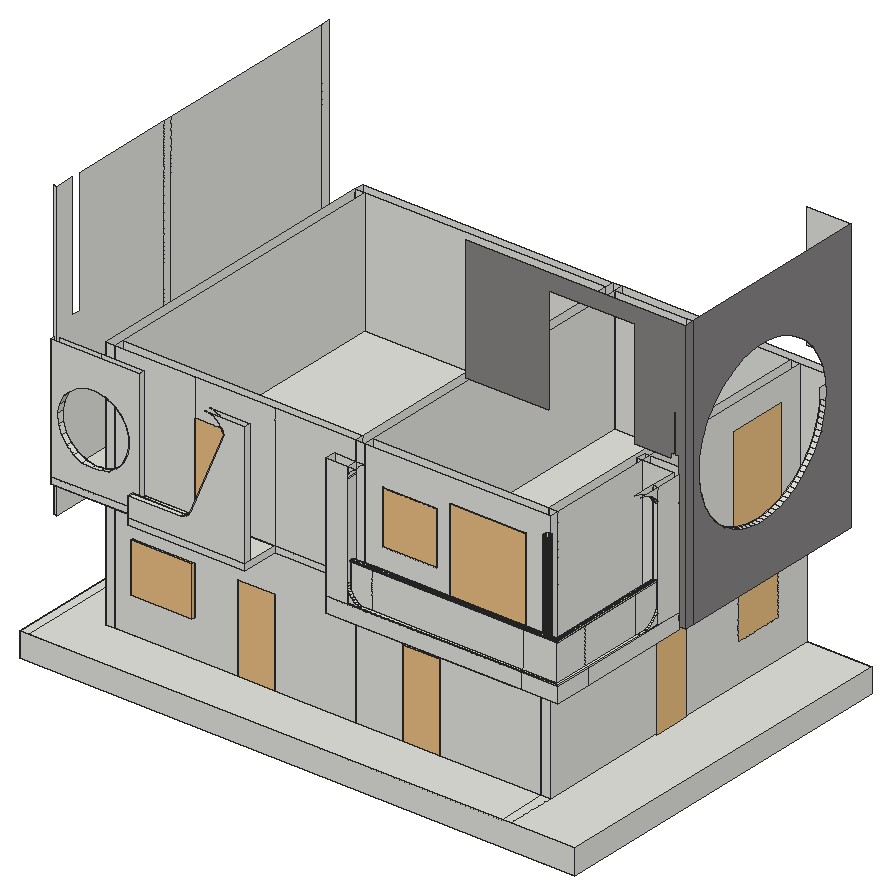
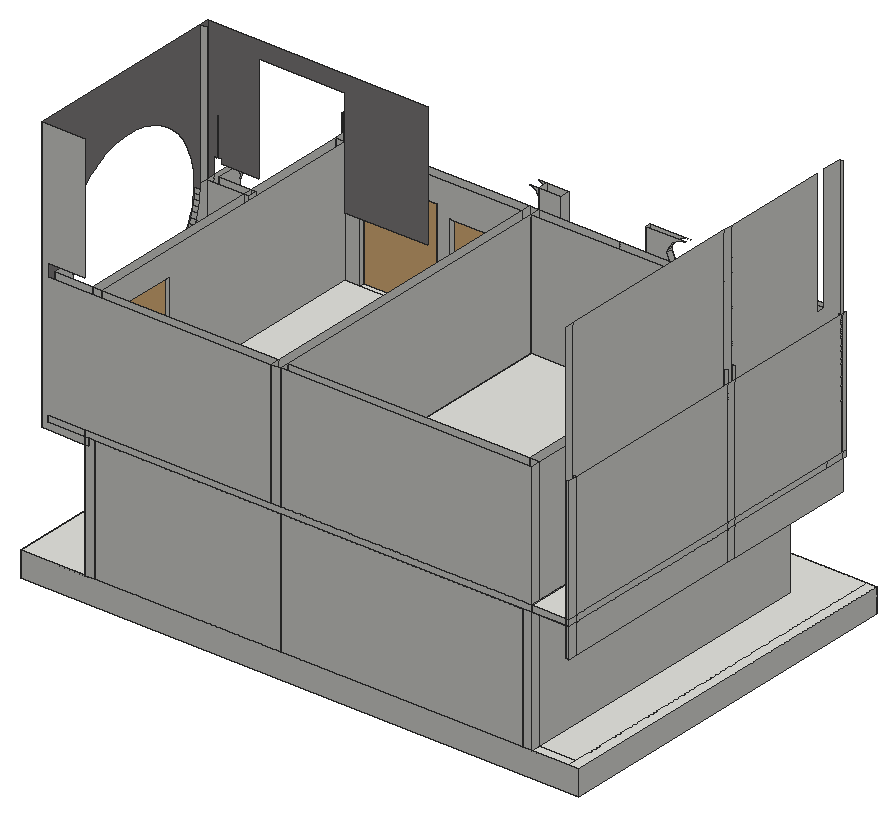
# SketchUp Ruby script. Lengths in inches.
U = 1.inch
M = Sketchup.active_model
def pt(a) = Geom::Point3d.new(a.map { |v| v * U })
def face(e, loops, mat)
  f = e.add_face(loops[0].map { |a| pt(a) })
  loops[1..].each { |l| e.add_face(l.map { |a| pt(a) }).erase! }
  f.material = f.back_material = mat if mat
  f
end
# faces: each face lists its corners as indices into pts; further lists are holes
def faces(e, pts, list, mat = nil) = list.each { |f| face(e, (f[0].is_a?(Array) ? f : [f]).map { |l| l.map { |i| pts[i] } }, mat) }
# xy, xz, yz: faces in a plane at the given z, y or x. An outline is a flat list of corners, or four numbers for a rectangle; further outlines are holes
def ring(l) = l.size == 4 ? [[l[0], l[1]], [l[2], l[1]], [l[2], l[3]], [l[0], l[3]]] : l.each_slice(2).to_a
def flat(e, list, mat, &to3) = list.each { |f| face(e, (f[0].is_a?(Array) ? f : [f]).map { |l| ring(l).map { |u, v| to3.(u, v) } }, mat) }
def xy(e, z, list, mat = nil) = flat(e, list, mat) { |x, y| [x, y, z] }
def xz(e, y, list, mat = nil) = flat(e, list, mat) { |x, z| [x, y, z] }
def yz(e, x, list, mat = nil) = flat(e, list, mat) { |y, z| [x, y, z] }
def lines(e, pts, list) = list.each { |a, b| e.add_line(pt(pts[a]), pt(pts[b])) }
# prism: a flat outline (further loops are holes) pulled along v
def prism(e, loops, v, mat = nil)
  f = face(e, loops, mat); d = Geom::Vector3d.new(v.map { |x| x * U })
  f.pushpull(f.normal.samedirection?(d) ? d.length : -d.length)
end
def box(e, o, s, mat = nil) = prism(e, [[o, [o[0] + s[0], o[1], o[2]], [o[0] + s[0], o[1] + s[1], o[2]], [o[0], o[1] + s[1], o[2]]]], [0, 0, s[2]], mat)
def at(x, y, z, deg = 0) = Geom::Transformation.translation(pt([x, y, z])) * Geom::Transformation.rotation(ORIGIN, Z_AXIS, deg.degrees)
def axes(o, x, y, z) = Geom::Transformation.new([*x, 0, *y, 0, *z, 0, *pt(o).to_a, 1])
def part(name) = M.definitions.add(name)
# library, detail: a bought-in or finely detailed component or shape, given as its bounding box
def library(name, o, s) = part(name).tap { |d| box(d.entities, o, s) }
def detail(e, o, s) = box(e.add_group.entities, o, s)
def put(e, d, t, mat = nil) = e.add_instance(d, t).tap { |i| i.material = mat if mat }
def group(e, t, mat = nil) = e.add_group.tap { |g| g.transformation = t; g.material = mat if mat }.entities
root = M.entities
M.materials.add("[Brick Tumbled]").color = [135, 132, 132]
c1 = library("Door 243 053",[-21.6,-2.79,-0.07],[43.2,5.58,82.64])
c2 = library("Window 46-08",[-34.875,-3.16,0],[69.74,4.26,70.87])
c3 = library("Window 46-47",[-61.02,-2.17,0],[122.04,4.34,74.02])
xy(root,-24,[[0,0,539.56,360]])
xy(root,0,[[0,0,9,360],[9,0,468,0,468,48,369.625,48,369.625,57,333.625,57,333.625,48,209.125,48,209.125,57,173.125,57,173.125,48,45,48,45,351,9,351],[468,0,477,48],[477,0,539.56,360],[45,48,54,360],
  [54,48,173.125,57],[209.125,48,288,57],[288,48,333.625,57],[369.625,48,468,57],[468,48,477,176.1875],
  [54,57,150,351],[150,57,159,351],[150,57,279,351],[159,57,279,351],[279,57,288,351],
  [288,57,468,351],[468,176.1875,477,212.1875],[468,212.1875,477,360],[9,351,45,360],[54,351,288,360],
  [288,351,468,360]])
xy(root,36,[[71,48,131,57],[468,276,477,324]])
xy(root,84,[[71,48,131,57],[173.125,48,209.125,57],[333.625,48,369.625,57],[468,176.1875,477,212.1875],[468,276,477,324]])
xy(root,91.5625,[[9,29.25,12.34,159.3125],[9,159.3125,12.34,168.3125],[9,168.3125,12.34,351],[9,351,12.34,360]])
xy(root,111.125,[[288,12,468,17.99],[468,12,477,17.99],[477,12,513,17.99],[509.76,17.99,513,48],[509.76,48,513,159.3125]])
xy(root,113.5,[[473.9375,159.3125,519.125,168.3125],[513,168.3125,513,351,473.75,351,473.75,360,519.125,360,519.125,168.3125]],"[Brick Tumbled]")
xy(root,120,[[95.3125,12,95.3125,25.8125,131,25.8125,131,48,209.125,48,209.125,12],[288,17.99,468,48],[468,17.99,477,48],[477,17.99,509.76,48],[9,25.8125,54,48],
  [54,25.8125,131,48],[9,48,45,351],[45,48,54,360],[54,48,288,57],[288,48,468,57],
  [468,48,477,48,477,159.3125,473.9375,159.3125,473.9375,168.3125,477,168.3125,477,351,473.75,351,473.75,360,468,360],[477,48,509.76,159.3125],[54,57,150,351],[150,57,159,351],[150,57,279,351],
  [279,57,288,351],[288,57,468,351],[473.9375,159.3125,477,168.3125],[477,159.3125,513,168.3125],[477,168.3125,513,351],
  [9,351,45,360],[54,351,288,360],[288,351,468,360],[473.75,351,477,360],[477,351,513,360]])
xy(root,126,[[95.3125,12,209.125,17.48],[288,12,308.6875,21.82],[308.6875,12,327.12,19.52],[327.12,12,327.12,19.52,505.48,19.52,505.48,159.3125,507.74,159.3125,507.74,112.72,513,112.72,513,12],[95.3125,17.48,209.125,17.48,209.125,48,131,48,131,25.8125,95.3125,25.8125],
  [[327.12,19.52,505.48,19.52,505.48,159.3125,477,159.3125,477,48,288,48,288,21.82,327.12,21.82],[493.53,20.08,492.64,20.28,491.83,20.7,491.16,21.32,490.67,22.09,490.39,22.96,490.35,23.875,490.55,24.77,490.98,25.58,491.59,26.25,492.37,26.74,493.24,27.01,494.15,27.05,495.04,26.85,495.85,26.43,496.52,25.8125,497.01,25.04,497.29,24.17,497.33,23.25,497.125,22.36,496.7,21.55,496.09,20.88,495.3125,20.39,494.44,20.12]],[308.6875,19.52,327.12,21.82],[493.53,20.08,492.64,20.28,491.83,20.7,491.16,21.32,490.67,22.09,490.39,22.96,490.35,23.875,490.55,24.77,490.98,25.58,491.59,26.25,492.37,26.74,493.24,27.01,494.15,27.05,495.04,26.85,495.85,26.43,496.52,25.8125,497.01,25.04,497.29,24.17,497.33,23.25,497.125,22.36,496.7,21.55,496.09,20.88,495.3125,20.39,494.44,20.12],[9,25.8125,54,31.1875],[54,25.8125,95.3125,31.1875],
  [95.3125,25.8125,131,25.8125,131,48,54,48,54,31.1875,95.3125,31.1875],[9,31.1875,54,48],[9,48,45,360],[45,48,54,351],[54,48,131,57],
  [131,48,173.125,57],[173.125,48,288,57],[288,48,297,360],[297,48,379.04,57],[379.04,48,453.36,57],
  [453.36,48,477,57],[54,57,288,351],[297,57,468,351],[468,57,468,269.23,477,269.23,477,168.3125,472.375,168.3125,472.375,159.3125,477,159.3125,477,57],[507.74,112.72,513,134.0625],
  [507.74,134.0625,513,134.0625,513,168.3125,477,168.3125,477,159.3125,507.74,159.3125],[472.375,159.3125,477,168.3125],[477,168.3125,513,351],[468,269.23,477,328.73],[468,328.73,477,351],
  [45,351,288,360],[297,351,477,360],[477,351,513,360]])
xy(root,127.25,[[308.6875,12,327.12,12,327.12,14.75,309.62,14.75,309.62,16.77,327.12,16.77,327.12,19.52,308.6875,19.52],[327.12,12,513,12,513,112.72,510.25,112.72,510.25,14.75,327.12,14.75],[309.62,14.75,327.12,16.77],[327.12,14.75,329.87,16.77],[329.87,14.75,329.87,16.77,508.23,16.77,508.23,109.97,510.25,109.97,510.25,14.75],
  [327.12,16.77,508.23,16.77,508.23,112.72,507.74,112.72,507.74,159.3125,505.48,159.3125,505.48,19.52,327.12,19.52],[508.23,109.97,510.25,112.72],[507.74,112.72,508.23,134.0625],[508.23,112.72,510.25,134.0625],[510.25,112.72,513,134.0625]])
xy(root,145.31,[[95.3125,12,145.3,17.48]])
xy(root,162.59,[[314.49,48,366.36,57]])
xy(root,163.25,[[[308.44,13.58,308.44,17.9375,507.0625,17.9375,507.0625,135.23,511.42,135.23,511.42,13.58],[309.62,14.75,510.25,14.75,510.25,134.0625,508.23,134.0625,508.23,16.77,309.62,16.77]],[309.62,14.75,309.62,16.77,508.23,16.77,508.23,134.0625,510.25,134.0625,510.25,14.75]])
xy(root,164.125,[[[308.44,13.58,511.42,13.58,511.42,135.23,507.0625,135.23,507.0625,17.9375,308.44,17.9375],[309.62,14.75,309.62,16.77,508.23,16.77,508.23,134.0625,510.25,134.0625,510.25,14.75]],[309.62,14.75,510.25,14.75,510.25,134.0625,508.23,134.0625,508.23,16.77,309.62,16.77]])
xy(root,210,[[131,48,173.125,57]])
xy(root,214.46,[[314.49,48,366.36,57]])
xy(root,222.27,[[468,269.23,477,328.73]])
xy(root,223.3125,[[379.04,48,453.36,57]])
xz(root,0,[[0,-24,539.56,0]])
xz(root,12,[[288,111.125,477,126],[477,111.125,513,126],[95.3125,120,209.125,126],[95.3125,126,209.125,126,209.125,246,170.0625,246,172.1875,245.88,174.28,245.51,176.32,244.91,178.28,244.08,180.13,243.03,181.84,241.77,183.41,240.33,184.79,238.71,185.98,236.95,186.96,235.07,187.72,233.08,188.25,231.02,155.44,151.72,154.86,150.87,154.22,150.06,153.52,149.29,152.77,148.59,151.96,147.94,151.11,147.36,150.21,146.84,149.28,146.38,148.32,146,147.33,145.7,146.32,145.46,145.3,145.31,95.3125,145.31],[288,126,308.6875,246],
  [308.6875,126,327.12,126,324.71,126.16,322.35,126.63,320.51,127.25,308.6875,127.25],[327.12,126,327.12,127.25,320.51,127.25,322.35,126.63,324.71,126.16],[327.12,126,477,127.25],[477,126,513,127.25],[308.6875,127.25,320.51,127.25,320.0625,127.4,317.9,128.47,315.9,129.81,314.09,131.4,312.5,133.21,311.16,135.21,310.09,137.375,309.32,139.66,308.85,142.02,308.6875,144.43],
  [308.6875,235.27,308.76,236.49,308.96,237.7,309.3,238.88,309.76,240.02,310.35,241.1,311.06,242.1,311.87,243.02,312.78,243.85,313.77,244.5625,314.84,245.17,315.97,245.65,317.15,246,308.6875,246]])
xz(root,13.58,[[308.44,163.25,329.87,164.125],[329.87,163.25,477,164.125],[477,163.25,511.42,164.125]])
xz(root,14.75,[[309.62,127.25,329.87,163.25],[329.87,127.25,477,163.25],[477,127.25,510.25,163.25],[309.62,163.25,329.87,164.125],[329.87,163.25,477,164.125],
  [477,163.25,510.25,164.125]])
xz(root,16.77,[[309.62,127.25,329.87,163.25],[329.87,127.25,477,163.25],[477,127.25,508.23,163.25],[309.62,163.25,329.87,164.125],[329.87,163.25,477,164.125],
  [477,163.25,508.23,164.125]])
xz(root,17.48,[[95.3125,126,95.3125,145.31,145.3,145.31,146.32,145.46,147.33,145.7,148.32,146,149.28,146.38,150.21,146.84,151.11,147.36,151.96,147.94,152.77,148.59,153.52,149.29,154.22,150.06,154.86,150.87,155.44,151.72,188.25,231.02,187.72,233.08,186.96,235.07,185.98,236.95,184.79,238.71,183.41,240.33,181.84,241.77,180.13,243.03,178.28,244.08,176.32,244.91,174.28,245.51,172.1875,245.88,170.0625,246,209.125,246,209.125,126]])
xz(root,17.9375,[[308.44,163.25,329.87,164.125],[329.87,163.25,477,164.125],[477,163.25,507.0625,164.125]])
xz(root,17.99,[[288,111.125,468,120],[468,111.125,477,120],[477,111.125,509.76,120]])
xz(root,19.52,[[308.6875,126,327.12,127.25],[327.12,126,477,127.25],[477,126,505.48,127.25]])
xz(root,21.82,[[288,126,308.6875,246],[308.6875,126,308.6875,144.43,308.85,142.02,309.32,139.66,310.09,137.375,311.16,135.21,312.5,133.21,314.09,131.4,315.9,129.81,317.9,128.47,320.0625,127.4,322.35,126.63,324.71,126.16,327.12,126],[308.6875,235.27,308.6875,246,317.15,246,315.97,245.65,314.84,245.17,313.77,244.5625,312.78,243.85,311.87,243.02,311.06,242.1,310.35,241.1,309.76,240.02,309.3,238.88,308.96,237.7,308.76,236.49]])
xz(root,25.8125,[[9,120,95.3125,126],[95.3125,120,131,126],[[9,126,95.3125,246],[48.3125,147.1,39.51,148.92,31.48,152.96,24.77,158.94,19.84,166.46,17.02,175,16.5,183.97,18.33,192.77,22.37,200.8,28.35,207.52,35.86,212.45,44.4,215.27,53.375,215.78,62.18,213.96,70.21,209.92,76.92,203.9375,81.85,196.42,84.67,187.88,85.1875,178.91,83.36,170.11,79.32,162.08,73.34,155.37,65.83,150.43,57.29,147.61]]])
xz(root,29.25,[[9,91.5625,12.34,378]])
xz(root,31.1875,[[9,126,9,246,54,246,54,215.66,53.375,215.78,44.4,215.27,35.86,212.45,28.35,207.52,22.37,200.8,18.33,192.77,16.5,183.97,17.02,175,19.84,166.46,24.77,158.94,31.48,152.96,39.51,148.92,48.3125,147.1,54,147.42,54,126],[54,126,54,147.42,57.29,147.61,65.83,150.43,73.34,155.37,79.32,162.08,83.36,170.11,85.1875,178.91,84.67,187.88,81.85,196.42,76.92,203.9375,70.21,209.92,62.18,213.96,54,215.66,54,246,95.3125,246,95.3125,126]])
xz(root,48,[[45,0,54,120],[[54,0,173.125,0,173.125,84,209.125,84,209.125,0,288,0,288,120,54,120],[71,36,131,84]],[288,0,333.625,0,333.625,84,369.625,84,369.625,0,468,0,468,120,288,120],[468,0,477,120],[9,120,45,126],
  [131,120,209.125,126],[209.125,120,288,126],[288,120,477,126],[45,126,54,246],[54,126,131,246],
  [173.125,126,209.125,126,209.125,246,131,246,131,210,173.125,210],[209.125,126,288,246],[288,126,297,246],[[297,126,379.04,126,379.04,223.3125,453.36,223.3125,453.36,126,477,126,477,246,297,246],[314.49,162.59,366.36,214.46]]])
xz(root,57,[[[54,0,150,120],[71,36,131,84]],[150,0,159,120],[159,0,159,120,279,120,279,0,209.125,0,209.125,84,173.125,84,173.125,0],[279,0,288,120],[288,0,288,120,468,120,468,0,369.625,0,369.625,84,333.625,84,333.625,0],
  [54,126,54,246,288,246,288,126,173.125,126,173.125,210,131,210,131,126],[[297,126,297,246,468,246,468,126,453.36,126,453.36,223.3125,379.04,223.3125,379.04,126],[314.49,162.59,366.36,214.46]],[468,126,477,246]])
xz(root,112.72,[[507.74,126,513,127.25]])
xz(root,134.0625,[[507.74,127.25,508.23,139.33],[508.23,127.25,510.25,139.33],[510.25,127.25,513,139.33],[507.74,139.33,508.23,139.33,508.23,164.125,510.25,164.125,510.25,139.33,513,139.33,513,231.76,507.74,231.76],[508.23,139.33,510.25,163.25],
  [508.23,163.25,510.25,164.125],[507.74,231.76,513,246]])
xz(root,135.23,[[507.0625,163.25,511.42,164.125]])
xz(root,159.3125,[[9,91.5625,12.34,258],[509.76,111.125,513,113.5],[509.76,113.5,513,120],[472.375,126,505.48,126,505.48,127.25,507.74,127.25,507.74,246,472.375,246],[505.48,126,507.74,127.25]])
xz(root,159.3125,[[513,113.5,519.125,113.5,519.125,378,306,378,306,258,386.17,258,386.17,361.875,469.61,361.875,469.61,258,505.25,258,505.25,262.3125,508.22,262.3125,508.22,298.9375,510.03,298.9375,510.03,262.3125,513,262.3125],[473.9375,113.5,509.76,120]],"[Brick Tumbled]")
xz(root,168.3125,[[9,91.5625,12.34,258],[473.9375,113.5,513,120],[513,113.5,519.125,378],[472.375,126,513,246]])
xz(root,176.1875,[[468,0,477,84]])
xz(root,212.1875,[[468,0,477,84]])
xz(root,269.23,[[468,126,477,222.27]])
xz(root,276,[[468,36,477,84]])
xz(root,324,[[468,36,477,84]])
xz(root,328.73,[[468,126,477,222.27]])
xz(root,351,[[54,0,150,120],[150,0,159,120],[159,0,279,120],[279,0,288,120],[288,0,468,120],
  [9,91.5625,12.34,120],[9,120,12.34,246],[45,126,54,246],[54,126,288,246],[297,126,468,246],
  [468,126,477,246],[477,126,513,246]])
xz(root,351,[[473.75,113.5,513,120]],"[Brick Tumbled]")
xz(root,360,[[0,-24,539.56,0],[45,0,54,120],[54,0,288,120],[288,0,468,120],[468,0,468,120,473.75,120,473.75,113.5,477,113.5,477,0],
  [9,91.5625,12.34,120],[477,113.5,477,120,513,120,513,126,297,126,297,246,513,246,513,258,477,258,477,378,519.125,378,519.125,113.5],[473.75,113.5,477,120],[9,120,12.34,126],[12.34,120,45,126],
  [45,120,477,126],[477,120,513,126],[9,126,12.34,246],[45,126,288,246],[288,126,297,246]])
yz(root,0,[[0,-24,360,0]])
yz(root,9,[[29.25,91.5625,159.3125,120],[159.3125,91.5625,168.3125,120],[168.3125,91.5625,351,120],[351,91.5625,360,120],[25.8125,120,29.25,126],
  [29.25,120,48,126],[48,120,159.3125,126],[159.3125,120,168.3125,126],[168.3125,120,351,126],[351,120,360,126],
  [25.8125,126,29.25,246],[29.25,126,31.1875,246],[31.1875,126,159.3125,246],[159.3125,126,168.3125,246],[168.3125,126,351,246],
  [351,126,360,246]])
yz(root,12.34,[[29.25,91.5625,159.3125,91.5625,159.3125,378,57,378,57,258,48,258,48,378,29.25,378],[159.3125,91.5625,168.3125,378],[168.3125,91.5625,351,378],[351,91.5625,360,378]])
yz(root,45,[[48,0,351,120],[351,0,360,120],[48,120,360,126],[48,126,351,246],[351,126,360,246]])
yz(root,54,[[48,0,57,120],[57,0,351,120],[351,0,360,120],[48,126,57,246],[57,126,351,246]])
yz(root,71,[[48,36,57,84]])
yz(root,95.3125,[[12,120,25.8125,126],[12,126,17.48,145.31],[25.8125,126,31.1875,246]])
yz(root,131,[[48,36,57,84],[25.8125,120,48,126],[48,126,57,210]])
yz(root,150,[[57,0,351,120]])
yz(root,159,[[57,0,351,120]])
yz(root,173.125,[[48,0,57,84],[48,126,57,210]])
yz(root,209.125,[[48,0,57,84],[12,120,48,126],[12,126,17.48,246]])
yz(root,279,[[57,0,351,120]])
yz(root,288,[[48,0,57,120],[57,0,351,120],[351,0,360,120],[12,111.125,12,126,48,126,48,120,17.99,120,17.99,111.125],[12,126,21.82,246],
  [48,126,57,246],[57,126,351,246],[351,126,360,246]])
yz(root,297,[[48,126,57,246],[57,126,351,246],[351,126,360,246]])
yz(root,308.44,[[13.58,163.25,17.9375,164.125]])
yz(root,308.6875,[[19.52,126,21.82,126,21.82,144.43,12,144.43,12,127.25,19.52,127.25],[12,144.43,21.82,235.27],[12,235.27,21.82,246]])
yz(root,309.62,[[14.75,127.25,16.77,163.25],[14.75,163.25,16.77,164.125]])
yz(root,314.49,[[48,162.59,57,214.46]])
yz(root,327.12,[[12,126,19.52,127.25]])
yz(root,333.625,[[48,0,57,84]])
yz(root,366.36,[[48,162.59,57,214.46]])
yz(root,369.625,[[48,0,57,84]])
yz(root,379.04,[[48,126,57,223.3125]])
yz(root,453.36,[[48,126,57,223.3125]])
yz(root,468,[[48,0,57,120],[[57,0,57,120,351,120,351,0,212.1875,0,212.1875,84,176.1875,84,176.1875,0],[276,36,324,84]],[351,0,360,120],[57,126,57,246,351,246,351,126,328.73,126,328.73,222.27,269.23,222.27,269.23,126]])
yz(root,472.375,[[159.3125,126,168.3125,246]])
yz(root,473.75,[[351,113.5,360,120]])
yz(root,473.9375,[[159.3125,113.5,168.3125,120]])
yz(root,477,[[[48,0,176.1875,0,176.1875,84,212.1875,84,212.1875,0,360,0,360,120,48,120],[276,36,324,84]],[48,120,360,126],[48,126,57,246],[57,126,269.23,126,269.23,222.27,328.73,222.27,328.73,126,351,126,351,246,57,246]])
yz(root,505.48,[[19.52,126,48,127.25],[48,126,159.3125,127.25]])
yz(root,507.0625,[[17.9375,163.25,48,164.125],[48,163.25,109.97,164.125],[109.97,163.25,135.23,164.125]])
yz(root,507.74,[[112.72,126,112.72,127.25,120.24,127.25,119.26,126.92,117.11,126.41,114.93,126.1],[112.72,126,114.93,126.1,117.11,126.41,119.26,126.92,120.24,127.25,134.0625,127.25,134.0625,126],[134.0625,126,159.3125,127.25],[120.24,127.25,121.36,127.625,123.375,128.52,125.3,129.61,127.12,130.86,128.8125,132.28,130.36,133.85,131.77,135.56,133,137.39,134.0625,139.33,134.0625,127.25],[134.0625,127.25,159.3125,246],
  [134.0625,231.76,133.07,233.81,131.875,235.75,130.5,237.57,128.95,239.25,127.25,240.77,125.41,242.12,123.45,243.28,121.38,244.25,119.23,245.01,117.02,245.56,114.76,245.89,112.49,246,134.0625,246]])
yz(root,508.23,[[16.77,127.25,48,163.25],[48,127.25,109.97,163.25],[109.97,127.25,134.0625,163.25],[16.77,163.25,48,164.125],[48,163.25,109.97,164.125],
  [109.97,163.25,134.0625,164.125]])
yz(root,509.76,[[17.99,111.125,48,120],[48,111.125,159.3125,120]])
yz(root,510.25,[[14.75,127.25,48,163.25],[48,127.25,109.97,163.25],[109.97,127.25,134.0625,163.25],[14.75,163.25,48,164.125],[48,163.25,109.97,164.125],
  [109.97,163.25,134.0625,164.125]])
yz(root,511.42,[[13.58,163.25,48,164.125],[48,163.25,109.97,164.125],[109.97,163.25,135.23,164.125]])
yz(root,513,[[12,111.125,48,126],[48,111.125,159.3125,126],[168.3125,113.5,351,120],[159.3125,120,168.3125,126],[168.3125,120,360,126],
  [12,126,48,127.25],[48,126,112.72,127.25],[112.72,126,114.93,126.1,117.11,126.41,119.26,126.92,120.24,127.25,112.72,127.25],[112.72,126,134.0625,126,134.0625,127.25,120.24,127.25,119.26,126.92,117.11,126.41,114.93,126.1],[134.0625,126,159.3125,246],
  [159.3125,126,168.3125,246],[168.3125,126,168.3125,246,175.45,246,175.42,245.46,175.47,240.59,175.82,235.72,176.48,230.89,177.45,226.11,178.71,221.4,180.26,216.78,182.1,212.26,184.22,207.87,186.62,203.62,189.27,199.53,192.18,195.62,195.32,191.89,198.7,188.37,202.29,185.07,206.08,182,210.05,179.17,214.19,176.6,218.49,174.29,222.92,172.26,227.48,170.51,232.13,169.06,236.87,167.89,241.66,167.03,246.51,166.46,251.38,166.21,256.25,166.26,261.12,166.61,265.95,167.27,270.73,168.24,275.44,169.5,280.0625,171.05,284.58,172.89,288.97,175.01,293.22,177.41,297.31,180.0625,301.23,182.97,304.95,186.11,308.47,189.49,311.77,193.08,314.84,196.87,317.67,200.84,320.24,204.98,322.55,209.28,324.58,213.71,326.33,218.27,327.79,222.92,328.95,227.65,329.81,232.45,330.375,237.3,330.63,242.17,330.59,246,351,246,351,126],[120.24,127.25,134.0625,127.25,134.0625,139.33,133,137.39,131.77,135.56,130.36,133.85,128.8125,132.28,127.12,130.86,125.3,129.61,123.375,128.52,121.36,127.625],[134.0625,231.76,134.0625,246,112.49,246,114.76,245.89,117.02,245.56,119.23,245.01,121.38,244.25,123.45,243.28,125.41,242.12,127.25,240.77,128.95,239.25,130.5,237.57,131.875,235.75,133.07,233.81]])
yz(root,519.125,[[159.3125,113.5,168.3125,378],[[168.3125,113.5,360,378],[251.38,166.21,246.51,166.46,241.66,167.03,236.87,167.89,232.13,169.06,227.48,170.51,222.92,172.26,218.49,174.29,214.19,176.6,210.05,179.17,206.08,182,202.29,185.07,198.7,188.37,195.32,191.89,192.18,195.62,189.27,199.53,186.62,203.62,184.22,207.87,182.1,212.26,180.26,216.78,178.71,221.4,177.45,226.11,176.48,230.89,175.82,235.72,175.47,240.59,175.42,245.46,175.67,250.33,176.24,255.18,177.1,259.98,178.27,264.71,179.73,269.36,181.47,273.92,183.51,278.35,185.8125,282.65,188.38,286.79,191.21,290.76,194.28,294.55,197.58,298.14,201.1,301.52,204.83,304.66,208.74,307.57,212.83,310.22,217.08,312.62,221.47,314.74,225.99,316.58,230.61,318.13,235.32,319.39,240.1,320.36,244.93,321.02,249.8,321.37,254.67,321.42,259.54,321.17,264.39,320.6,269.1875,319.74,273.92,318.57,278.57,317.12,283.125,315.37,287.56,313.33,291.86,311.03,296,308.46,299.97,305.63,303.76,302.5625,307.35,299.26,310.73,295.74,313.87,292.01,316.78,288.1,319.43,284.01,321.83,279.76,323.95,275.37,325.79,270.85,327.34,266.23,328.6,261.52,329.57,256.74,330.23,251.91,330.58,247.04,330.63,242.17,330.375,237.3,329.81,232.45,328.95,227.65,327.79,222.92,326.33,218.27,324.58,213.71,322.55,209.28,320.24,204.98,317.67,200.84,314.84,196.87,311.77,193.08,308.47,189.49,304.95,186.11,301.23,182.97,297.31,180.0625,293.22,177.41,288.97,175.01,284.58,172.89,280.0625,171.05,275.44,169.5,270.73,168.24,265.95,167.27,261.12,166.61,256.25,166.26]]],"[Brick Tumbled]")
yz(root,539.56,[[0,-24,360,0]])
p = [[324.71,12,126.16],[327.12,12,126],[327.12,19.52,126],[327.12,21.82,126],[324.71,21.82,126.16],[492.64,20.28,126],
  [493.53,20.08,126],[493.53,20.08,246],[492.64,20.28,246],[494.44,20.12,126],[494.44,20.12,246],[495.3125,20.39,126],
  [495.3125,20.39,246],[491.83,20.7,126],[491.83,20.7,246],[496.09,20.88,126],[496.09,20.88,246],[491.16,21.32,126],
  [491.16,21.32,246],[496.7,21.55,126],[496.7,21.55,246],[490.67,22.09,126],[490.67,22.09,246],[497.125,22.36,126],
  [497.125,22.36,246],[490.39,22.96,126],[490.39,22.96,246],[497.33,23.25,126],[497.33,23.25,246],[490.35,23.875,126],
  [490.35,23.875,246],[497.29,24.17,126],[497.29,24.17,246],[490.55,24.77,126],[490.55,24.77,246],[497.01,25.04,126],
  [497.01,25.04,246],[490.98,25.58,126],[490.98,25.58,246],[496.52,25.8125,126],[496.52,25.8125,246],[491.59,26.25,126],
  [491.59,26.25,246],[495.85,26.43,126],[495.85,26.43,246],[492.37,26.74,126],[492.37,26.74,246],[495.04,26.85,126],
  [495.04,26.85,246],[493.24,27.01,126],[493.24,27.01,246],[494.15,27.05,126],[494.15,27.05,246],[513,112.72,126],
  [513,114.93,126.1],[507.74,114.93,126.1],[507.74,112.72,126],[513,117.11,126.41],[507.74,117.11,126.41],[322.35,12,126.63],
  [322.35,21.82,126.63],[513,119.26,126.92],[507.74,119.26,126.92],[320.51,12,127.25],[320.0625,21.82,127.4],[320.0625,12,127.4],
  [513,120.24,127.25],[513,121.36,127.625],[507.74,121.36,127.625],[507.74,120.24,127.25],[317.9,12,128.47],[317.9,21.82,128.47],
  [513,123.375,128.52],[507.74,123.375,128.52],[315.9,12,129.81],[315.9,21.82,129.81],[513,125.3,129.61],[507.74,125.3,129.61],
  [513,127.12,130.86],[507.74,127.12,130.86],[314.09,12,131.4],[314.09,21.82,131.4],[513,128.8125,132.28],[507.74,128.8125,132.28],
  [312.5,12,133.21],[312.5,21.82,133.21],[513,130.36,133.85],[507.74,130.36,133.85],[311.16,12,135.21],[311.16,21.82,135.21],
  [513,131.77,135.56],[507.74,131.77,135.56],[310.09,12,137.375],[310.09,21.82,137.375],[513,133,137.39],[507.74,133,137.39],
  [309.32,12,139.66],[309.32,21.82,139.66],[513,134.0625,139.33],[510.25,134.0625,139.33],[508.23,134.0625,139.33],[507.74,134.0625,139.33],
  [308.85,12,142.02],[308.85,21.82,142.02],[308.6875,12,144.43],[308.6875,21.82,144.43],[145.3,12,145.31],[146.32,12,145.46],
  [146.32,17.48,145.46],[145.3,17.48,145.31],[147.33,12,145.7],[147.33,17.48,145.7],[148.32,12,146],[148.32,17.48,146],
  [149.28,12,146.38],[149.28,17.48,146.38],[150.21,12,146.84],[150.21,17.48,146.84],[151.11,12,147.36],[151.11,17.48,147.36],
  [39.51,25.8125,148.92],[48.3125,25.8125,147.1],[48.3125,31.1875,147.1],[39.51,31.1875,148.92],[57.29,25.8125,147.61],[57.29,31.1875,147.61],
  [54,31.1875,147.42],[151.96,12,147.94],[151.96,17.48,147.94],[65.83,25.8125,150.43],[65.83,31.1875,150.43],[152.77,12,148.59],
  [152.77,17.48,148.59],[153.52,12,149.29],[153.52,17.48,149.29],[31.48,25.8125,152.96],[31.48,31.1875,152.96],[154.22,12,150.06],
  [154.22,17.48,150.06],[154.86,12,150.87],[154.86,17.48,150.87],[73.34,25.8125,155.37],[73.34,31.1875,155.37],[155.44,12,151.72],
  [155.44,17.48,151.72],[188.25,12,231.02],[188.25,17.48,231.02],[24.77,25.8125,158.94],[24.77,31.1875,158.94],[79.32,25.8125,162.08],
  [79.32,31.1875,162.08],[19.84,25.8125,166.46],[19.84,31.1875,166.46],[83.36,25.8125,170.11],[83.36,31.1875,170.11],[519.125,246.51,166.46],
  [519.125,251.38,166.21],[513,251.38,166.21],[513,246.51,166.46],[519.125,256.25,166.26],[513,256.25,166.26],[519.125,261.12,166.61],
  [513,261.12,166.61],[17.02,25.8125,175],[17.02,31.1875,175],[519.125,241.66,167.03],[513,241.66,167.03],[519.125,265.95,167.27],
  [513,265.95,167.27],[519.125,236.87,167.89],[513,236.87,167.89],[519.125,270.73,168.24],[513,270.73,168.24],[519.125,232.13,169.06],
  [513,232.13,169.06],[519.125,275.44,169.5],[513,275.44,169.5],[519.125,227.48,170.51],[513,227.48,170.51],[519.125,280.0625,171.05],
  [513,280.0625,171.05],[85.1875,25.8125,178.91],[85.1875,31.1875,178.91],[519.125,222.92,172.26],[513,222.92,172.26],[519.125,284.58,172.89],
  [513,284.58,172.89],[519.125,218.49,174.29],[513,218.49,174.29],[519.125,288.97,175.01],[513,288.97,175.01],[519.125,214.19,176.6],
  [513,214.19,176.6],[16.5,25.8125,183.97],[16.5,31.1875,183.97],[519.125,293.22,177.41],[513,293.22,177.41],[519.125,210.05,179.17],
  [513,210.05,179.17],[519.125,297.31,180.0625],[513,297.31,180.0625],[84.67,25.8125,187.88],[84.67,31.1875,187.88],[519.125,206.08,182],
  [513,206.08,182],[519.125,301.23,182.97],[513,301.23,182.97],[519.125,202.29,185.07],[513,202.29,185.07],[519.125,304.95,186.11],
  [513,304.95,186.11],[18.33,25.8125,192.77],[18.33,31.1875,192.77],[519.125,198.7,188.37],[513,198.7,188.37],[519.125,308.47,189.49],
  [513,308.47,189.49],[81.85,25.8125,196.42],[81.85,31.1875,196.42],[519.125,195.32,191.89],[513,195.32,191.89],[519.125,311.77,193.08],
  [513,311.77,193.08],[519.125,192.18,195.62],[513,192.18,195.62],[22.37,25.8125,200.8],[22.37,31.1875,200.8],[519.125,314.84,196.87],
  [513,314.84,196.87],[519.125,189.27,199.53],[513,189.27,199.53],[76.92,25.8125,203.9375],[76.92,31.1875,203.9375],[519.125,317.67,200.84],
  [513,317.67,200.84],[519.125,186.62,203.62],[513,186.62,203.62],[28.35,25.8125,207.52],[28.35,31.1875,207.52],[519.125,320.24,204.98],
  [513,320.24,204.98],[519.125,184.22,207.87],[513,184.22,207.87],[70.21,25.8125,209.92],[70.21,31.1875,209.92],[519.125,322.55,209.28],
  [513,322.55,209.28],[35.86,25.8125,212.45],[35.86,31.1875,212.45],[519.125,182.1,212.26],[513,182.1,212.26],[519.125,324.58,213.71],
  [513,324.58,213.71],[62.18,25.8125,213.96],[62.18,31.1875,213.96],[519.125,180.26,216.78],[513,180.26,216.78],[44.4,25.8125,215.27],
  [44.4,31.1875,215.27],[519.125,326.33,218.27],[513,326.33,218.27],[53.375,25.8125,215.78],[53.375,31.1875,215.78],[54,31.1875,215.66],
  [519.125,178.71,221.4],[513,178.71,221.4],[519.125,327.79,222.92],[513,327.79,222.92],[519.125,177.45,226.11],[513,177.45,226.11],
  [519.125,328.95,227.65],[513,328.95,227.65],[519.125,176.48,230.89],[513,176.48,230.89],[519.125,329.81,232.45],[513,329.81,232.45],
  [519.125,175.82,235.72],[513,175.82,235.72],[187.72,12,233.08],[187.72,17.48,233.08],[513,134.0625,231.76],[513,133.07,233.81],
  [507.74,133.07,233.81],[507.74,134.0625,231.76],[519.125,330.375,237.3],[513,330.375,237.3],[186.96,12,235.07],[186.96,17.48,235.07],
  [513,131.875,235.75],[507.74,131.875,235.75],[185.98,12,236.95],[185.98,17.48,236.95],[308.76,12,236.49],[308.6875,12,235.27],
  [308.6875,21.82,235.27],[308.76,21.82,236.49],[519.125,175.47,240.59],[513,175.47,240.59],[513,130.5,237.57],[507.74,130.5,237.57]]
faces(root,p,[[0,1,2,3,4],[5,6,7,8],[6,9,10,7],[9,11,12,10],[13,5,8,14],[11,15,16,12],[17,13,14,18],[15,19,20,16],
  [21,17,18,22],[19,23,24,20],[25,21,22,26],[23,27,28,24],[29,25,26,30],[27,31,32,28],[33,29,30,34],[31,35,36,32],
  [37,33,34,38],[35,39,40,36],[41,37,38,42],[39,43,44,40],[45,41,42,46],[43,47,48,44],[49,45,46,50],[47,51,52,48],
  [51,49,50,52],[53,54,55,56],[54,57,58,55],[59,0,4,60],[57,61,62,58],[63,59,60,64,65],[61,66,67,68,69,62],[70,65,64,71],
  [67,72,73,68],[74,70,71,75],[72,76,77,73],[76,78,79,77],[80,74,75,81],[78,82,83,79],[84,80,81,85],[82,86,87,83],
  [88,84,85,89],[86,90,91,87],[92,88,89,93],[90,94,95,91],[96,92,93,97],[94,98,99,100,101,95],[102,96,97,103],[104,102,103,105],
  [106,107,108,109],[107,110,111,108],[110,112,113,111],[112,114,115,113],[114,116,117,115],[116,118,119,117],[120,121,122,123],[121,124,125,126,122],
  [118,127,128,119],[124,129,130,125],[127,131,132,128],[131,133,134,132],[135,120,123,136],[133,137,138,134],[137,139,140,138],[129,141,142,130],
  [139,143,144,140],[143,145,146,144],[147,135,136,148],[141,149,150,142],[151,147,148,152],[149,153,154,150],[155,156,157,158],[156,159,160,157],
  [159,161,162,160],[163,151,152,164],[165,155,158,166],[161,167,168,162],[169,165,166,170],[167,171,172,168],[173,169,170,174],[171,175,176,172],
  [177,173,174,178],[175,179,180,176],[153,181,182,154],[183,177,178,184],[179,185,186,180],[187,183,184,188],[185,189,190,186],[191,187,188,192],
  [193,163,164,194],[189,195,196,190],[197,191,192,198],[195,199,200,196],[181,201,202,182],[203,197,198,204],[199,205,206,200],[207,203,204,208],
  [205,209,210,206],[211,193,194,212],[213,207,208,214],[209,215,216,210],[201,217,218,202],[219,213,214,220],[215,221,222,216],[223,219,220,224],
  [225,211,212,226],[221,227,228,222],[229,223,224,230],[217,231,232,218],[227,233,234,228],[235,229,230,236],[237,225,226,238],[233,239,240,234],
  [241,235,236,242],[231,243,244,232],[239,245,246,240],[247,237,238,248],[249,241,242,250],[245,251,252,246],[243,253,254,244],[255,249,250,256],
  [257,247,248,258],[251,259,260,252],[253,261,262,263,254],[261,257,258,262],[264,255,256,265],[259,266,267,260],[268,264,265,269],[266,270,271,267],
  [272,268,269,273],[270,274,275,271],[276,272,273,277],[145,278,279,146],[280,281,282,283],[274,284,285,275],[278,286,287,279],[281,288,289,282],
  [286,290,291,287],[292,293,294,295],[296,276,277,297],[288,298,299,289]])
put(root,c1,axes([475.09,193.92,-0.5625],[0,0.83329,0],[-1,0,0],[0,0,1.01657]))
put(root,c1,axes([351.625,50.79,0.07],[0.83329,0,0],[0,1,0],[0,0,1.01657]))
put(root,c1,axes([191.125,50.79,0.07],[0.83329,0,0],[0,1,0],[0,0,1.01657]))
put(root,c2,axes([100.96,48.62,35.97],[0.86027,0,0],[0,1,0],[0,0,0.67733]))
put(root,c2,axes([473.84,300,36],[0,0.68821,0],[-1,0,0],[0,0,0.67733]))
put(root,c1,axes([152.0625,50.79,126.07],[0.97506,0,0],[0,1,0],[0,0,1.01657]))
put(root,c3,axes([416.2,50.17,126],[0.60888,0,0],[0,1,0],[0,0,1.29702]))
put(root,c2,axes([473.84,298.98,126],[0,0.8531,0],[-1,0,0],[0,0,1.35852]))
put(root,c2,axes([340.43,51.16,162.59],[0.74377,0,0],[0,1,0],[0,0,0.72475]))
